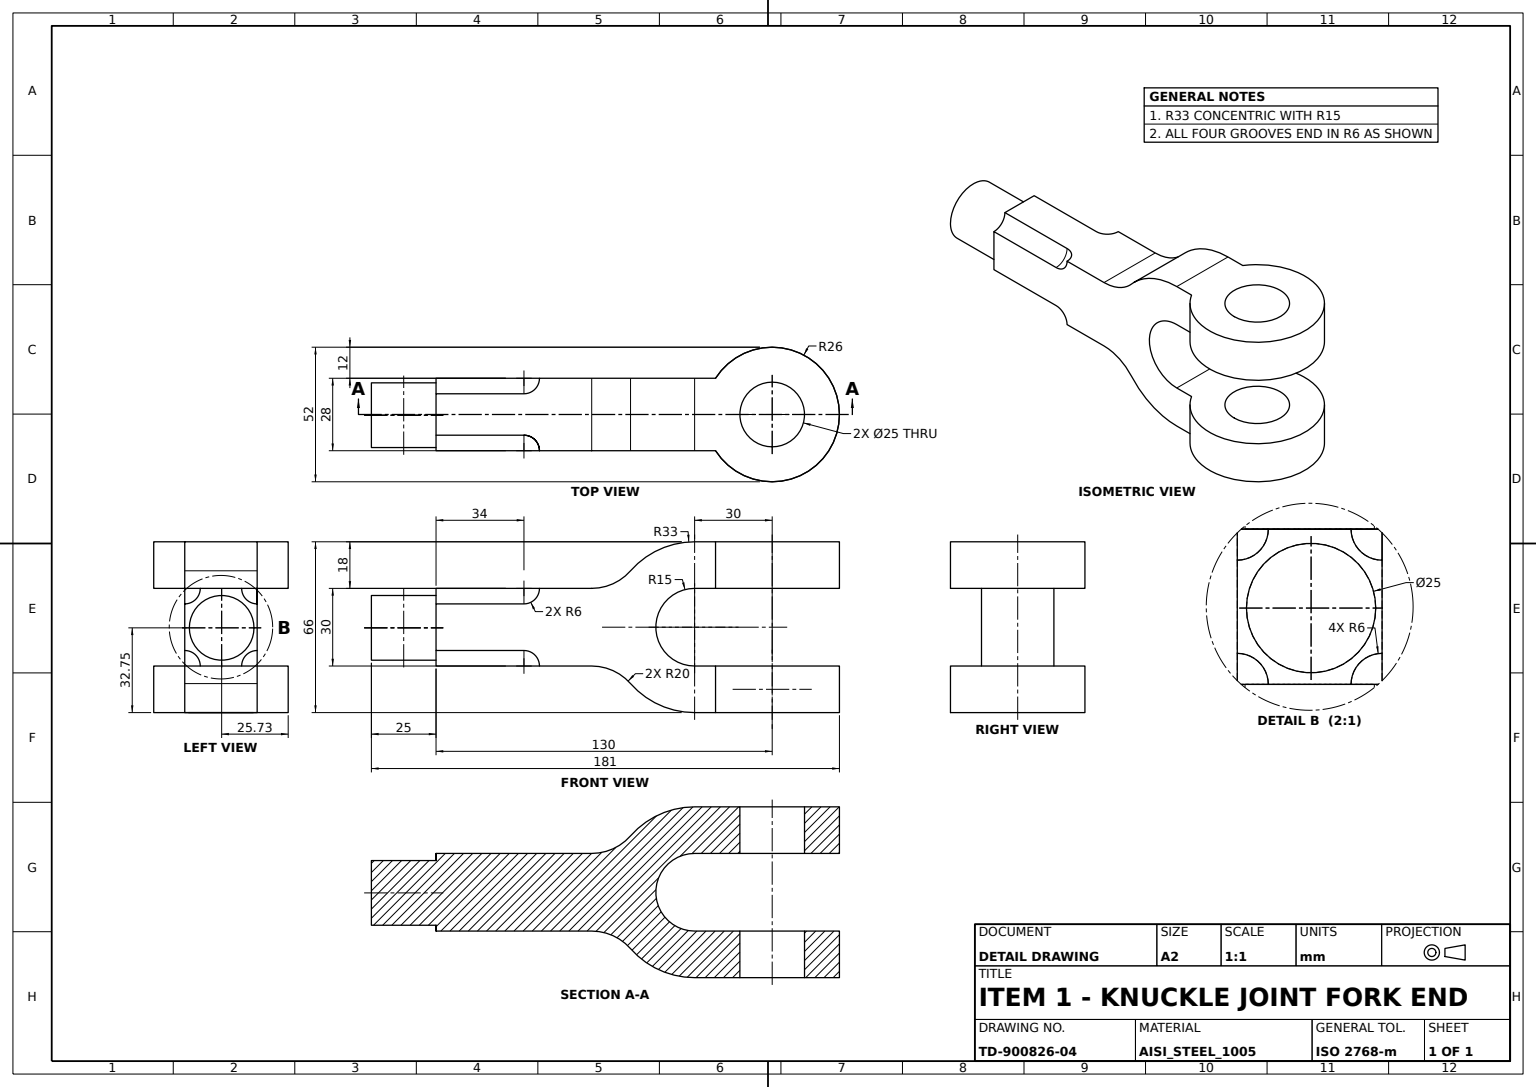
ISO-10303-21;
HEADER;
FILE_DESCRIPTION((''),'2;1');
FILE_NAME('','',(''),(''),'','','');
FILE_SCHEMA(('AUTOMOTIVE_DESIGN'));
ENDSEC;
DATA;
#1=APPLICATION_CONTEXT('');
#2=PRODUCT_CONTEXT('',#1,'mechanical');
#3=PRODUCT('','','',(#2));
#4=PRODUCT_DEFINITION_FORMATION('','',#3);
#5=PRODUCT_DEFINITION_CONTEXT('',#1,'design');
#6=PRODUCT_DEFINITION('','',#4,#5);
#7=PRODUCT_DEFINITION_SHAPE('','',#6);
#8=(LENGTH_UNIT()NAMED_UNIT(*)SI_UNIT(.MILLI.,.METRE.));
#9=(NAMED_UNIT(*)PLANE_ANGLE_UNIT()SI_UNIT($,.RADIAN.));
#10=(NAMED_UNIT(*)SI_UNIT($,.STERADIAN.)SOLID_ANGLE_UNIT());
#11=UNCERTAINTY_MEASURE_WITH_UNIT(LENGTH_MEASURE(0.005),#8,'distance_accuracy_value','');
#12=(GEOMETRIC_REPRESENTATION_CONTEXT(3)GLOBAL_UNCERTAINTY_ASSIGNED_CONTEXT((#11))GLOBAL_UNIT_ASSIGNED_CONTEXT((#8,#9,#10))REPRESENTATION_CONTEXT('',''));
#13=CARTESIAN_POINT('',(12.772907,-155.,-0.250667));
#14=VERTEX_POINT('',#13);
#15=CARTESIAN_POINT('',(0.272907,-155.,-0.250667));
#16=DIRECTION('',(0.,-1.,0.));
#17=DIRECTION('',(1.,0.,0.));
#18=AXIS2_PLACEMENT_3D('',#15,#16,#17);
#19=CIRCLE('',#18,12.5);
#20=EDGE_CURVE('',#14,#14,#19,.T.);
#21=ORIENTED_EDGE('',*,*,#20,.T.);
#22=EDGE_LOOP('',(#21));
#23=FACE_BOUND('',#22,.T.);
#24=DIRECTION('',(0.,0.,-1.));
#25=AXIS2_PLACEMENT_3D('',#15,#16,#24);
#26=PLANE('',#25);
#27=ADVANCED_FACE('',(#23),#26,.T.);
#28=CARTESIAN_POINT('',(14.,-30.,-15.));
#29=VERTEX_POINT('',#28);
#30=CARTESIAN_POINT('',(14.,-30.,15.));
#31=VERTEX_POINT('',#30);
#32=CARTESIAN_POINT('',(14.,-30.,0.));
#33=DIRECTION('',(-1.,0.,0.));
#34=DIRECTION('',(0.,1.,0.));
#35=AXIS2_PLACEMENT_3D('',#32,#33,#34);
#36=CIRCLE('',#35,15.);
#37=EDGE_CURVE('',#29,#31,#36,.T.);
#38=ORIENTED_EDGE('',*,*,#37,.F.);
#39=CARTESIAN_POINT('',(-14.,-30.,-15.));
#40=VERTEX_POINT('',#39);
#41=VECTOR('',#33,1000.);
#42=LINE('',#28,#41);
#43=EDGE_CURVE('',#29,#40,#42,.T.);
#44=ORIENTED_EDGE('',*,*,#43,.T.);
#45=CARTESIAN_POINT('',(-14.,-30.,15.));
#46=VERTEX_POINT('',#45);
#47=CARTESIAN_POINT('',(-14.,-30.,0.));
#48=AXIS2_PLACEMENT_3D('',#47,#33,#34);
#49=CIRCLE('',#48,15.);
#50=EDGE_CURVE('',#40,#46,#49,.T.);
#51=ORIENTED_EDGE('',*,*,#50,.T.);
#52=LINE('',#30,#41);
#53=EDGE_CURVE('',#31,#46,#52,.T.);
#54=ORIENTED_EDGE('',*,*,#53,.F.);
#55=EDGE_LOOP('',(#38,#44,#51,#54));
#56=FACE_BOUND('',#55,.T.);
#57=DIRECTION('',(0.,0.,1.));
#58=AXIS2_PLACEMENT_3D('',#32,#33,#57);
#59=CYLINDRICAL_SURFACE('',#58,15.);
#60=ADVANCED_FACE('',(#56),#59,.F.);
#61=CARTESIAN_POINT('',(-14.,-69.799497,-15.));
#62=VERTEX_POINT('',#61);
#63=CARTESIAN_POINT('',(-14.,-90.,-15.));
#64=VERTEX_POINT('',#63);
#65=CARTESIAN_POINT('',(-14.,54870.,-15.));
#66=VECTOR('',#16,1000.);
#67=LINE('',#65,#66);
#68=EDGE_CURVE('',#62,#64,#67,.T.);
#69=ORIENTED_EDGE('',*,*,#68,.F.);
#70=CARTESIAN_POINT('',(14.,-69.799497,-15.));
#71=VERTEX_POINT('',#70);
#72=VECTOR('',#17,1000.);
#73=LINE('',#70,#72);
#74=EDGE_CURVE('',#62,#71,#73,.T.);
#75=ORIENTED_EDGE('',*,*,#74,.T.);
#76=CARTESIAN_POINT('',(14.,-90.,-15.));
#77=VERTEX_POINT('',#76);
#78=CARTESIAN_POINT('',(14.,54870.,-15.));
#79=LINE('',#78,#66);
#80=EDGE_CURVE('',#71,#77,#79,.T.);
#81=ORIENTED_EDGE('',*,*,#80,.T.);
#82=CARTESIAN_POINT('',(8.,-96.,-15.));
#83=VERTEX_POINT('',#82);
#84=CARTESIAN_POINT('',(14.,-96.,-15.));
#85=AXIS2_PLACEMENT_3D('',#84,#57,#17);
#86=CIRCLE('',#85,6.);
#87=EDGE_CURVE('',#77,#83,#86,.T.);
#88=ORIENTED_EDGE('',*,*,#87,.T.);
#89=CARTESIAN_POINT('',(8.,-130.,-15.));
#90=VERTEX_POINT('',#89);
#91=CARTESIAN_POINT('',(8.,-90.,-15.));
#92=LINE('',#91,#66);
#93=EDGE_CURVE('',#83,#90,#92,.T.);
#94=ORIENTED_EDGE('',*,*,#93,.T.);
#95=CARTESIAN_POINT('',(-8.,-130.,-15.));
#96=VERTEX_POINT('',#95);
#97=CARTESIAN_POINT('',(14.,-130.,-15.));
#98=LINE('',#97,#41);
#99=EDGE_CURVE('',#90,#96,#98,.T.);
#100=ORIENTED_EDGE('',*,*,#99,.T.);
#101=CARTESIAN_POINT('',(-8.,-96.,-15.));
#102=VERTEX_POINT('',#101);
#103=CARTESIAN_POINT('',(-8.,-90.,-15.));
#104=LINE('',#103,#66);
#105=EDGE_CURVE('',#102,#96,#104,.T.);
#106=ORIENTED_EDGE('',*,*,#105,.F.);
#107=CARTESIAN_POINT('',(-14.,-96.,-15.));
#108=AXIS2_PLACEMENT_3D('',#107,#57,#17);
#109=CIRCLE('',#108,6.);
#110=EDGE_CURVE('',#102,#64,#109,.T.);
#111=ORIENTED_EDGE('',*,*,#110,.T.);
#112=EDGE_LOOP('',(#69,#75,#81,#88,#94,#100,#106,#111));
#113=FACE_BOUND('',#112,.T.);
#114=AXIS2_PLACEMENT_3D('',#78,#57,#17);
#115=PLANE('',#114);
#116=ADVANCED_FACE('',(#113),#115,.F.);
#117=CARTESIAN_POINT('',(-14.,-21.908902,-15.));
#118=VERTEX_POINT('',#117);
#119=CARTESIAN_POINT('',(-14.,-20.5,-15.));
#120=LINE('',#119,#66);
#121=EDGE_CURVE('',#118,#40,#120,.T.);
#122=ORIENTED_EDGE('',*,*,#121,.T.);
#123=ORIENTED_EDGE('',*,*,#43,.F.);
#124=CARTESIAN_POINT('',(14.,-21.908902,-15.));
#125=VERTEX_POINT('',#124);
#126=CARTESIAN_POINT('',(14.,-20.5,-15.));
#127=LINE('',#126,#66);
#128=EDGE_CURVE('',#125,#29,#127,.T.);
#129=ORIENTED_EDGE('',*,*,#128,.F.);
#130=CARTESIAN_POINT('',(0.,0.,-15.));
#131=AXIS2_PLACEMENT_3D('',#130,#57,#17);
#132=CIRCLE('',#131,26.);
#133=EDGE_CURVE('',#125,#118,#132,.T.);
#134=ORIENTED_EDGE('',*,*,#133,.T.);
#135=EDGE_LOOP('',(#122,#123,#129,#134));
#136=FACE_BOUND('',#135,.T.);
#137=CARTESIAN_POINT('',(12.5,0.,-15.));
#138=VERTEX_POINT('',#137);
#139=CIRCLE('',#131,12.5);
#140=EDGE_CURVE('',#138,#138,#139,.T.);
#141=ORIENTED_EDGE('',*,*,#140,.F.);
#142=EDGE_LOOP('',(#141));
#143=FACE_BOUND('',#142,.T.);
#144=AXIS2_PLACEMENT_3D('',#126,#24,#33);
#145=PLANE('',#144);
#146=ADVANCED_FACE('',(#136,#143),#145,.F.);
#147=CARTESIAN_POINT('',(14.,-21.908902,33.));
#148=VERTEX_POINT('',#147);
#149=CARTESIAN_POINT('',(14.,-30.,33.));
#150=VERTEX_POINT('',#149);
#151=CARTESIAN_POINT('',(14.,-20.5,33.));
#152=LINE('',#151,#66);
#153=EDGE_CURVE('',#148,#150,#152,.T.);
#154=ORIENTED_EDGE('',*,*,#153,.F.);
#155=CARTESIAN_POINT('',(-14.,-21.908902,33.));
#156=VERTEX_POINT('',#155);
#157=CARTESIAN_POINT('',(0.,0.,33.));
#158=AXIS2_PLACEMENT_3D('',#157,#57,#17);
#159=CIRCLE('',#158,26.);
#160=EDGE_CURVE('',#148,#156,#159,.T.);
#161=ORIENTED_EDGE('',*,*,#160,.T.);
#162=CARTESIAN_POINT('',(-14.,-30.,33.));
#163=VERTEX_POINT('',#162);
#164=CARTESIAN_POINT('',(-14.,-20.5,33.));
#165=LINE('',#164,#66);
#166=EDGE_CURVE('',#156,#163,#165,.T.);
#167=ORIENTED_EDGE('',*,*,#166,.T.);
#168=LINE('',#149,#41);
#169=EDGE_CURVE('',#150,#163,#168,.T.);
#170=ORIENTED_EDGE('',*,*,#169,.F.);
#171=EDGE_LOOP('',(#154,#161,#167,#170));
#172=FACE_BOUND('',#171,.T.);
#173=CARTESIAN_POINT('',(12.5,0.,33.));
#174=VERTEX_POINT('',#173);
#175=CIRCLE('',#158,12.5);
#176=EDGE_CURVE('',#174,#174,#175,.T.);
#177=ORIENTED_EDGE('',*,*,#176,.F.);
#178=EDGE_LOOP('',(#177));
#179=FACE_BOUND('',#178,.T.);
#180=AXIS2_PLACEMENT_3D('',#151,#24,#33);
#181=PLANE('',#180);
#182=ADVANCED_FACE('',(#172,#179),#181,.F.);
#183=CARTESIAN_POINT('',(-14.,-96.,-9.));
#184=VERTEX_POINT('',#183);
#185=AXIS2_PLACEMENT_3D('',#107,#17,#24);
#186=CIRCLE('',#185,6.);
#187=EDGE_CURVE('',#64,#184,#186,.T.);
#188=ORIENTED_EDGE('',*,*,#187,.T.);
#189=CARTESIAN_POINT('',(-14.,-130.,-9.));
#190=VERTEX_POINT('',#189);
#191=CARTESIAN_POINT('',(-14.,-90.,-9.));
#192=LINE('',#191,#66);
#193=EDGE_CURVE('',#184,#190,#192,.T.);
#194=ORIENTED_EDGE('',*,*,#193,.T.);
#195=CARTESIAN_POINT('',(-14.,-130.,9.));
#196=VERTEX_POINT('',#195);
#197=CARTESIAN_POINT('',(-14.,-130.,-15.));
#198=VECTOR('',#57,1000.);
#199=LINE('',#197,#198);
#200=EDGE_CURVE('',#190,#196,#199,.T.);
#201=ORIENTED_EDGE('',*,*,#200,.T.);
#202=CARTESIAN_POINT('',(-14.,-96.,9.));
#203=VERTEX_POINT('',#202);
#204=CARTESIAN_POINT('',(-14.,-90.,9.));
#205=LINE('',#204,#66);
#206=EDGE_CURVE('',#203,#196,#205,.T.);
#207=ORIENTED_EDGE('',*,*,#206,.F.);
#208=CARTESIAN_POINT('',(-14.,-90.,15.));
#209=VERTEX_POINT('',#208);
#210=CARTESIAN_POINT('',(-14.,-96.,15.));
#211=AXIS2_PLACEMENT_3D('',#210,#17,#24);
#212=CIRCLE('',#211,6.);
#213=EDGE_CURVE('',#203,#209,#212,.T.);
#214=ORIENTED_EDGE('',*,*,#213,.T.);
#215=CARTESIAN_POINT('',(-14.,-69.799497,15.));
#216=VERTEX_POINT('',#215);
#217=CARTESIAN_POINT('',(-14.,54870.,15.));
#218=LINE('',#217,#66);
#219=EDGE_CURVE('',#216,#209,#218,.T.);
#220=ORIENTED_EDGE('',*,*,#219,.F.);
#221=CARTESIAN_POINT('',(-14.,-54.780819,21.792453));
#222=VERTEX_POINT('',#221);
#223=CARTESIAN_POINT('',(-14.,-69.799497,35.));
#224=AXIS2_PLACEMENT_3D('',#223,#17,#24);
#225=CIRCLE('',#224,20.);
#226=EDGE_CURVE('',#216,#222,#225,.T.);
#227=ORIENTED_EDGE('',*,*,#226,.T.);
#228=AXIS2_PLACEMENT_3D('',#47,#17,#34);
#229=CIRCLE('',#228,33.);
#230=EDGE_CURVE('',#163,#222,#229,.T.);
#231=ORIENTED_EDGE('',*,*,#230,.F.);
#232=ORIENTED_EDGE('',*,*,#166,.F.);
#233=CARTESIAN_POINT('',(-14.,-21.908902,15.));
#234=VERTEX_POINT('',#233);
#235=VECTOR('',#24,1000.);
#236=LINE('',#155,#235);
#237=EDGE_CURVE('',#234,#156,#236,.F.);
#238=ORIENTED_EDGE('',*,*,#237,.F.);
#239=VECTOR('',#34,1000.);
#240=LINE('',#45,#239);
#241=EDGE_CURVE('',#46,#234,#240,.T.);
#242=ORIENTED_EDGE('',*,*,#241,.F.);
#243=ORIENTED_EDGE('',*,*,#50,.F.);
#244=ORIENTED_EDGE('',*,*,#121,.F.);
#245=CARTESIAN_POINT('',(-14.,-21.908902,-33.));
#246=VERTEX_POINT('',#245);
#247=LINE('',#245,#198);
#248=EDGE_CURVE('',#118,#246,#247,.F.);
#249=ORIENTED_EDGE('',*,*,#248,.T.);
#250=CARTESIAN_POINT('',(-14.,-30.,-33.));
#251=VERTEX_POINT('',#250);
#252=LINE('',#250,#239);
#253=EDGE_CURVE('',#251,#246,#252,.T.);
#254=ORIENTED_EDGE('',*,*,#253,.F.);
#255=CARTESIAN_POINT('',(-14.,-54.780819,-21.792453));
#256=VERTEX_POINT('',#255);
#257=EDGE_CURVE('',#256,#251,#229,.T.);
#258=ORIENTED_EDGE('',*,*,#257,.F.);
#259=CARTESIAN_POINT('',(-14.,-69.799497,-35.));
#260=AXIS2_PLACEMENT_3D('',#259,#17,#24);
#261=CIRCLE('',#260,20.);
#262=EDGE_CURVE('',#256,#62,#261,.T.);
#263=ORIENTED_EDGE('',*,*,#262,.T.);
#264=ORIENTED_EDGE('',*,*,#68,.T.);
#265=EDGE_LOOP('',(#188,#194,#201,#207,#214,#220,#227,#231,#232,#238,#242,#243,#244,#249,#254,#258,#263,#264));
#266=FACE_BOUND('',#265,.T.);
#267=AXIS2_PLACEMENT_3D('',#47,#17,#24);
#268=PLANE('',#267);
#269=ADVANCED_FACE('',(#266),#268,.F.);
#270=CARTESIAN_POINT('',(14.,-21.908902,15.));
#271=VERTEX_POINT('',#270);
#272=LINE('',#147,#235);
#273=EDGE_CURVE('',#271,#148,#272,.F.);
#274=ORIENTED_EDGE('',*,*,#273,.T.);
#275=ORIENTED_EDGE('',*,*,#153,.T.);
#276=CARTESIAN_POINT('',(14.,-54.780819,21.792453));
#277=VERTEX_POINT('',#276);
#278=AXIS2_PLACEMENT_3D('',#32,#17,#34);
#279=CIRCLE('',#278,33.);
#280=EDGE_CURVE('',#150,#277,#279,.T.);
#281=ORIENTED_EDGE('',*,*,#280,.T.);
#282=CARTESIAN_POINT('',(14.,-69.799497,15.));
#283=VERTEX_POINT('',#282);
#284=CARTESIAN_POINT('',(14.,-69.799497,35.));
#285=AXIS2_PLACEMENT_3D('',#284,#17,#24);
#286=CIRCLE('',#285,20.);
#287=EDGE_CURVE('',#277,#283,#286,.F.);
#288=ORIENTED_EDGE('',*,*,#287,.T.);
#289=CARTESIAN_POINT('',(14.,-90.,15.));
#290=VERTEX_POINT('',#289);
#291=CARTESIAN_POINT('',(14.,54870.,15.));
#292=LINE('',#291,#66);
#293=EDGE_CURVE('',#283,#290,#292,.T.);
#294=ORIENTED_EDGE('',*,*,#293,.T.);
#295=CARTESIAN_POINT('',(14.,-96.,9.));
#296=VERTEX_POINT('',#295);
#297=CARTESIAN_POINT('',(14.,-96.,15.));
#298=AXIS2_PLACEMENT_3D('',#297,#17,#24);
#299=CIRCLE('',#298,6.);
#300=EDGE_CURVE('',#290,#296,#299,.F.);
#301=ORIENTED_EDGE('',*,*,#300,.T.);
#302=CARTESIAN_POINT('',(14.,-130.,9.));
#303=VERTEX_POINT('',#302);
#304=CARTESIAN_POINT('',(14.,-90.,9.));
#305=LINE('',#304,#66);
#306=EDGE_CURVE('',#296,#303,#305,.T.);
#307=ORIENTED_EDGE('',*,*,#306,.T.);
#308=CARTESIAN_POINT('',(14.,-130.,-9.));
#309=VERTEX_POINT('',#308);
#310=CARTESIAN_POINT('',(14.,-130.,15.));
#311=LINE('',#310,#235);
#312=EDGE_CURVE('',#303,#309,#311,.T.);
#313=ORIENTED_EDGE('',*,*,#312,.T.);
#314=CARTESIAN_POINT('',(14.,-96.,-9.));
#315=VERTEX_POINT('',#314);
#316=CARTESIAN_POINT('',(14.,-90.,-9.));
#317=LINE('',#316,#66);
#318=EDGE_CURVE('',#315,#309,#317,.T.);
#319=ORIENTED_EDGE('',*,*,#318,.F.);
#320=AXIS2_PLACEMENT_3D('',#84,#17,#24);
#321=CIRCLE('',#320,6.);
#322=EDGE_CURVE('',#315,#77,#321,.F.);
#323=ORIENTED_EDGE('',*,*,#322,.T.);
#324=ORIENTED_EDGE('',*,*,#80,.F.);
#325=CARTESIAN_POINT('',(14.,-54.780819,-21.792453));
#326=VERTEX_POINT('',#325);
#327=CARTESIAN_POINT('',(14.,-69.799497,-35.));
#328=AXIS2_PLACEMENT_3D('',#327,#17,#24);
#329=CIRCLE('',#328,20.);
#330=EDGE_CURVE('',#71,#326,#329,.F.);
#331=ORIENTED_EDGE('',*,*,#330,.T.);
#332=CARTESIAN_POINT('',(14.,-30.,-33.));
#333=VERTEX_POINT('',#332);
#334=EDGE_CURVE('',#326,#333,#279,.T.);
#335=ORIENTED_EDGE('',*,*,#334,.T.);
#336=CARTESIAN_POINT('',(14.,-21.908902,-33.));
#337=VERTEX_POINT('',#336);
#338=LINE('',#332,#239);
#339=EDGE_CURVE('',#333,#337,#338,.T.);
#340=ORIENTED_EDGE('',*,*,#339,.T.);
#341=LINE('',#336,#198);
#342=EDGE_CURVE('',#125,#337,#341,.F.);
#343=ORIENTED_EDGE('',*,*,#342,.F.);
#344=ORIENTED_EDGE('',*,*,#128,.T.);
#345=ORIENTED_EDGE('',*,*,#37,.T.);
#346=LINE('',#30,#239);
#347=EDGE_CURVE('',#31,#271,#346,.T.);
#348=ORIENTED_EDGE('',*,*,#347,.T.);
#349=EDGE_LOOP('',(#274,#275,#281,#288,#294,#301,#307,#313,#319,#323,#324,#331,#335,#340,#343,#344,#345,#348));
#350=FACE_BOUND('',#349,.T.);
#351=AXIS2_PLACEMENT_3D('',#32,#17,#24);
#352=PLANE('',#351);
#353=ADVANCED_FACE('',(#350),#352,.T.);
#354=ORIENTED_EDGE('',*,*,#300,.F.);
#355=CARTESIAN_POINT('',(8.,-96.,15.));
#356=VERTEX_POINT('',#355);
#357=AXIS2_PLACEMENT_3D('',#297,#24,#33);
#358=CIRCLE('',#357,6.);
#359=EDGE_CURVE('',#356,#290,#358,.T.);
#360=ORIENTED_EDGE('',*,*,#359,.F.);
#361=AXIS2_PLACEMENT_3D('',#297,#16,#24);
#362=CIRCLE('',#361,6.);
#363=EDGE_CURVE('',#296,#356,#362,.F.);
#364=ORIENTED_EDGE('',*,*,#363,.F.);
#365=EDGE_LOOP('',(#354,#360,#364));
#366=FACE_BOUND('',#365,.T.);
#367=SPHERICAL_SURFACE('',#361,6.);
#368=ADVANCED_FACE('',(#366),#367,.F.);
#369=LINE('',#325,#41);
#370=EDGE_CURVE('',#326,#256,#369,.T.);
#371=ORIENTED_EDGE('',*,*,#370,.T.);
#372=ORIENTED_EDGE('',*,*,#257,.T.);
#373=LINE('',#332,#41);
#374=EDGE_CURVE('',#333,#251,#373,.T.);
#375=ORIENTED_EDGE('',*,*,#374,.F.);
#376=ORIENTED_EDGE('',*,*,#334,.F.);
#377=EDGE_LOOP('',(#371,#372,#375,#376));
#378=FACE_BOUND('',#377,.T.);
#379=CYLINDRICAL_SURFACE('',#58,33.);
#380=ADVANCED_FACE('',(#378),#379,.T.);
#381=CARTESIAN_POINT('',(0.,0.,-33.));
#382=AXIS2_PLACEMENT_3D('',#381,#57,#17);
#383=CIRCLE('',#382,26.);
#384=EDGE_CURVE('',#337,#246,#383,.T.);
#385=ORIENTED_EDGE('',*,*,#384,.T.);
#386=ORIENTED_EDGE('',*,*,#248,.F.);
#387=ORIENTED_EDGE('',*,*,#133,.F.);
#388=ORIENTED_EDGE('',*,*,#342,.T.);
#389=EDGE_LOOP('',(#385,#386,#387,#388));
#390=FACE_BOUND('',#389,.T.);
#391=CYLINDRICAL_SURFACE('',#382,26.);
#392=ADVANCED_FACE('',(#390),#391,.T.);
#393=ORIENTED_EDGE('',*,*,#87,.F.);
#394=ORIENTED_EDGE('',*,*,#322,.F.);
#395=AXIS2_PLACEMENT_3D('',#84,#16,#24);
#396=CIRCLE('',#395,6.);
#397=EDGE_CURVE('',#83,#315,#396,.F.);
#398=ORIENTED_EDGE('',*,*,#397,.F.);
#399=EDGE_LOOP('',(#393,#394,#398));
#400=FACE_BOUND('',#399,.T.);
#401=AXIS2_PLACEMENT_3D('',#84,#34,#57);
#402=SPHERICAL_SURFACE('',#401,6.);
#403=ADVANCED_FACE('',(#400),#402,.F.);
#404=ORIENTED_EDGE('',*,*,#280,.F.);
#405=ORIENTED_EDGE('',*,*,#169,.T.);
#406=ORIENTED_EDGE('',*,*,#230,.T.);
#407=LINE('',#276,#41);
#408=EDGE_CURVE('',#222,#277,#407,.F.);
#409=ORIENTED_EDGE('',*,*,#408,.T.);
#410=EDGE_LOOP('',(#404,#405,#406,#409));
#411=FACE_BOUND('',#410,.T.);
#412=ADVANCED_FACE('',(#411),#379,.T.);
#413=AXIS2_PLACEMENT_3D('',#107,#16,#24);
#414=CIRCLE('',#413,6.);
#415=EDGE_CURVE('',#184,#102,#414,.F.);
#416=ORIENTED_EDGE('',*,*,#415,.T.);
#417=ORIENTED_EDGE('',*,*,#105,.T.);
#418=AXIS2_PLACEMENT_3D('',#197,#34,#17);
#419=CIRCLE('',#418,6.);
#420=EDGE_CURVE('',#190,#96,#419,.T.);
#421=ORIENTED_EDGE('',*,*,#420,.F.);
#422=ORIENTED_EDGE('',*,*,#193,.F.);
#423=EDGE_LOOP('',(#416,#417,#421,#422));
#424=FACE_BOUND('',#423,.T.);
#425=AXIS2_PLACEMENT_3D('',#63,#16,#24);
#426=CYLINDRICAL_SURFACE('',#425,6.);
#427=ADVANCED_FACE('',(#424),#426,.F.);
#428=ORIENTED_EDGE('',*,*,#415,.F.);
#429=ORIENTED_EDGE('',*,*,#187,.F.);
#430=ORIENTED_EDGE('',*,*,#110,.F.);
#431=EDGE_LOOP('',(#428,#429,#430));
#432=FACE_BOUND('',#431,.T.);
#433=AXIS2_PLACEMENT_3D('',#107,#34,#57);
#434=SPHERICAL_SURFACE('',#433,6.);
#435=ADVANCED_FACE('',(#432),#434,.F.);
#436=CARTESIAN_POINT('',(8.,-130.,15.));
#437=VERTEX_POINT('',#436);
#438=CARTESIAN_POINT('',(8.,-90.,15.));
#439=LINE('',#438,#66);
#440=EDGE_CURVE('',#356,#437,#439,.T.);
#441=ORIENTED_EDGE('',*,*,#440,.F.);
#442=ORIENTED_EDGE('',*,*,#359,.T.);
#443=ORIENTED_EDGE('',*,*,#293,.F.);
#444=LINE('',#215,#72);
#445=EDGE_CURVE('',#283,#216,#444,.F.);
#446=ORIENTED_EDGE('',*,*,#445,.T.);
#447=ORIENTED_EDGE('',*,*,#219,.T.);
#448=CARTESIAN_POINT('',(-8.,-96.,15.));
#449=VERTEX_POINT('',#448);
#450=AXIS2_PLACEMENT_3D('',#210,#24,#33);
#451=CIRCLE('',#450,6.);
#452=EDGE_CURVE('',#209,#449,#451,.T.);
#453=ORIENTED_EDGE('',*,*,#452,.T.);
#454=CARTESIAN_POINT('',(-8.,-130.,15.));
#455=VERTEX_POINT('',#454);
#456=CARTESIAN_POINT('',(-8.,-90.,15.));
#457=LINE('',#456,#66);
#458=EDGE_CURVE('',#449,#455,#457,.T.);
#459=ORIENTED_EDGE('',*,*,#458,.T.);
#460=CARTESIAN_POINT('',(-14.,-130.,15.));
#461=LINE('',#460,#72);
#462=EDGE_CURVE('',#455,#437,#461,.T.);
#463=ORIENTED_EDGE('',*,*,#462,.T.);
#464=EDGE_LOOP('',(#441,#442,#443,#446,#447,#453,#459,#463));
#465=FACE_BOUND('',#464,.T.);
#466=AXIS2_PLACEMENT_3D('',#217,#24,#33);
#467=PLANE('',#466);
#468=ADVANCED_FACE('',(#465),#467,.F.);
#469=CARTESIAN_POINT('',(12.5,0.,-33.));
#470=VERTEX_POINT('',#469);
#471=CIRCLE('',#382,12.5);
#472=EDGE_CURVE('',#470,#470,#471,.T.);
#473=ORIENTED_EDGE('',*,*,#472,.F.);
#474=EDGE_LOOP('',(#473));
#475=FACE_BOUND('',#474,.T.);
#476=ORIENTED_EDGE('',*,*,#140,.T.);
#477=EDGE_LOOP('',(#476));
#478=FACE_BOUND('',#477,.T.);
#479=CYLINDRICAL_SURFACE('',#382,12.5);
#480=ADVANCED_FACE('',(#475,#478),#479,.F.);
#481=ORIENTED_EDGE('',*,*,#213,.F.);
#482=AXIS2_PLACEMENT_3D('',#210,#16,#24);
#483=CIRCLE('',#482,6.);
#484=EDGE_CURVE('',#449,#203,#483,.F.);
#485=ORIENTED_EDGE('',*,*,#484,.F.);
#486=ORIENTED_EDGE('',*,*,#452,.F.);
#487=EDGE_LOOP('',(#481,#485,#486));
#488=FACE_BOUND('',#487,.T.);
#489=AXIS2_PLACEMENT_3D('',#210,#34,#57);
#490=SPHERICAL_SURFACE('',#489,6.);
#491=ADVANCED_FACE('',(#488),#490,.F.);
#492=ORIENTED_EDGE('',*,*,#176,.T.);
#493=EDGE_LOOP('',(#492));
#494=FACE_BOUND('',#493,.T.);
#495=CARTESIAN_POINT('',(12.5,0.,15.));
#496=VERTEX_POINT('',#495);
#497=CARTESIAN_POINT('',(0.,0.,15.));
#498=AXIS2_PLACEMENT_3D('',#497,#57,#17);
#499=CIRCLE('',#498,12.5);
#500=EDGE_CURVE('',#496,#496,#499,.T.);
#501=ORIENTED_EDGE('',*,*,#500,.F.);
#502=EDGE_LOOP('',(#501));
#503=FACE_BOUND('',#502,.T.);
#504=AXIS2_PLACEMENT_3D('',#157,#24,#33);
#505=CYLINDRICAL_SURFACE('',#504,12.5);
#506=ADVANCED_FACE('',(#494,#503),#505,.F.);
#507=AXIS2_PLACEMENT_3D('',#97,#34,#17);
#508=CIRCLE('',#507,6.);
#509=EDGE_CURVE('',#90,#309,#508,.T.);
#510=ORIENTED_EDGE('',*,*,#509,.F.);
#511=ORIENTED_EDGE('',*,*,#93,.F.);
#512=ORIENTED_EDGE('',*,*,#397,.T.);
#513=ORIENTED_EDGE('',*,*,#318,.T.);
#514=EDGE_LOOP('',(#510,#511,#512,#513));
#515=FACE_BOUND('',#514,.T.);
#516=AXIS2_PLACEMENT_3D('',#76,#16,#24);
#517=CYLINDRICAL_SURFACE('',#516,6.);
#518=ADVANCED_FACE('',(#515),#517,.F.);
#519=ORIENTED_EDGE('',*,*,#472,.T.);
#520=EDGE_LOOP('',(#519));
#521=FACE_BOUND('',#520,.T.);
#522=ORIENTED_EDGE('',*,*,#339,.F.);
#523=ORIENTED_EDGE('',*,*,#374,.T.);
#524=ORIENTED_EDGE('',*,*,#253,.T.);
#525=ORIENTED_EDGE('',*,*,#384,.F.);
#526=EDGE_LOOP('',(#522,#523,#524,#525));
#527=FACE_BOUND('',#526,.T.);
#528=AXIS2_PLACEMENT_3D('',#332,#57,#17);
#529=PLANE('',#528);
#530=ADVANCED_FACE('',(#521,#527),#529,.F.);
#531=CARTESIAN_POINT('',(12.772907,-130.,-0.250667));
#532=VERTEX_POINT('',#531);
#533=CARTESIAN_POINT('',(0.272907,-130.,-0.250667));
#534=AXIS2_PLACEMENT_3D('',#533,#16,#17);
#535=CIRCLE('',#534,12.5);
#536=EDGE_CURVE('',#532,#532,#535,.T.);
#537=ORIENTED_EDGE('',*,*,#536,.F.);
#538=EDGE_LOOP('',(#537));
#539=FACE_BOUND('',#538,.T.);
#540=ORIENTED_EDGE('',*,*,#312,.F.);
#541=AXIS2_PLACEMENT_3D('',#310,#16,#17);
#542=CIRCLE('',#541,6.);
#543=EDGE_CURVE('',#437,#303,#542,.T.);
#544=ORIENTED_EDGE('',*,*,#543,.F.);
#545=ORIENTED_EDGE('',*,*,#462,.F.);
#546=AXIS2_PLACEMENT_3D('',#460,#34,#17);
#547=CIRCLE('',#546,6.);
#548=EDGE_CURVE('',#455,#196,#547,.T.);
#549=ORIENTED_EDGE('',*,*,#548,.T.);
#550=ORIENTED_EDGE('',*,*,#200,.F.);
#551=ORIENTED_EDGE('',*,*,#420,.T.);
#552=ORIENTED_EDGE('',*,*,#99,.F.);
#553=ORIENTED_EDGE('',*,*,#509,.T.);
#554=EDGE_LOOP('',(#540,#544,#545,#549,#550,#551,#552,#553));
#555=FACE_BOUND('',#554,.T.);
#556=CARTESIAN_POINT('',(0.,-130.,0.));
#557=AXIS2_PLACEMENT_3D('',#556,#34,#57);
#558=PLANE('',#557);
#559=ADVANCED_FACE('',(#539,#555),#558,.F.);
#560=ORIENTED_EDGE('',*,*,#536,.T.);
#561=EDGE_LOOP('',(#560));
#562=FACE_BOUND('',#561,.T.);
#563=ORIENTED_EDGE('',*,*,#20,.F.);
#564=EDGE_LOOP('',(#563));
#565=FACE_BOUND('',#564,.T.);
#566=AXIS2_PLACEMENT_3D('',#15,#34,#57);
#567=CYLINDRICAL_SURFACE('',#566,12.5);
#568=ADVANCED_FACE('',(#562,#565),#567,.T.);
#569=ORIENTED_EDGE('',*,*,#287,.F.);
#570=ORIENTED_EDGE('',*,*,#408,.F.);
#571=ORIENTED_EDGE('',*,*,#226,.F.);
#572=ORIENTED_EDGE('',*,*,#445,.F.);
#573=EDGE_LOOP('',(#569,#570,#571,#572));
#574=FACE_BOUND('',#573,.T.);
#575=AXIS2_PLACEMENT_3D('',#284,#33,#57);
#576=CYLINDRICAL_SURFACE('',#575,20.);
#577=ADVANCED_FACE('',(#574),#576,.F.);
#578=ORIENTED_EDGE('',*,*,#363,.T.);
#579=ORIENTED_EDGE('',*,*,#440,.T.);
#580=ORIENTED_EDGE('',*,*,#543,.T.);
#581=ORIENTED_EDGE('',*,*,#306,.F.);
#582=EDGE_LOOP('',(#578,#579,#580,#581));
#583=FACE_BOUND('',#582,.T.);
#584=AXIS2_PLACEMENT_3D('',#289,#16,#24);
#585=CYLINDRICAL_SURFACE('',#584,6.);
#586=ADVANCED_FACE('',(#583),#585,.F.);
#587=ORIENTED_EDGE('',*,*,#500,.T.);
#588=EDGE_LOOP('',(#587));
#589=FACE_BOUND('',#588,.T.);
#590=ORIENTED_EDGE('',*,*,#347,.F.);
#591=ORIENTED_EDGE('',*,*,#53,.T.);
#592=ORIENTED_EDGE('',*,*,#241,.T.);
#593=CIRCLE('',#498,26.);
#594=EDGE_CURVE('',#271,#234,#593,.T.);
#595=ORIENTED_EDGE('',*,*,#594,.F.);
#596=EDGE_LOOP('',(#590,#591,#592,#595));
#597=FACE_BOUND('',#596,.T.);
#598=AXIS2_PLACEMENT_3D('',#30,#57,#17);
#599=PLANE('',#598);
#600=ADVANCED_FACE('',(#589,#597),#599,.F.);
#601=ORIENTED_EDGE('',*,*,#160,.F.);
#602=ORIENTED_EDGE('',*,*,#273,.F.);
#603=ORIENTED_EDGE('',*,*,#594,.T.);
#604=ORIENTED_EDGE('',*,*,#237,.T.);
#605=EDGE_LOOP('',(#601,#602,#603,#604));
#606=FACE_BOUND('',#605,.T.);
#607=CYLINDRICAL_SURFACE('',#504,26.);
#608=ADVANCED_FACE('',(#606),#607,.T.);
#609=ORIENTED_EDGE('',*,*,#370,.F.);
#610=ORIENTED_EDGE('',*,*,#330,.F.);
#611=ORIENTED_EDGE('',*,*,#74,.F.);
#612=ORIENTED_EDGE('',*,*,#262,.F.);
#613=EDGE_LOOP('',(#609,#610,#611,#612));
#614=FACE_BOUND('',#613,.T.);
#615=AXIS2_PLACEMENT_3D('',#327,#33,#57);
#616=CYLINDRICAL_SURFACE('',#615,20.);
#617=ADVANCED_FACE('',(#614),#616,.F.);
#618=ORIENTED_EDGE('',*,*,#548,.F.);
#619=ORIENTED_EDGE('',*,*,#458,.F.);
#620=ORIENTED_EDGE('',*,*,#484,.T.);
#621=ORIENTED_EDGE('',*,*,#206,.T.);
#622=EDGE_LOOP('',(#618,#619,#620,#621));
#623=FACE_BOUND('',#622,.T.);
#624=AXIS2_PLACEMENT_3D('',#208,#16,#24);
#625=CYLINDRICAL_SURFACE('',#624,6.);
#626=ADVANCED_FACE('',(#623),#625,.F.);
#627=CLOSED_SHELL('',(#27,#60,#116,#146,#182,#269,#353,#368,#380,#392,#403,#412,#427,#435,#468,#480,#491,#506,#518,#530,#559,#568,#577,#586,#600,#608,#617,#626));
#628=MANIFOLD_SOLID_BREP('',#627);
#629=ADVANCED_BREP_SHAPE_REPRESENTATION('',(#628),#12);
#630=SHAPE_DEFINITION_REPRESENTATION(#7,#629);
ENDSEC;
END-ISO-10303-21;
